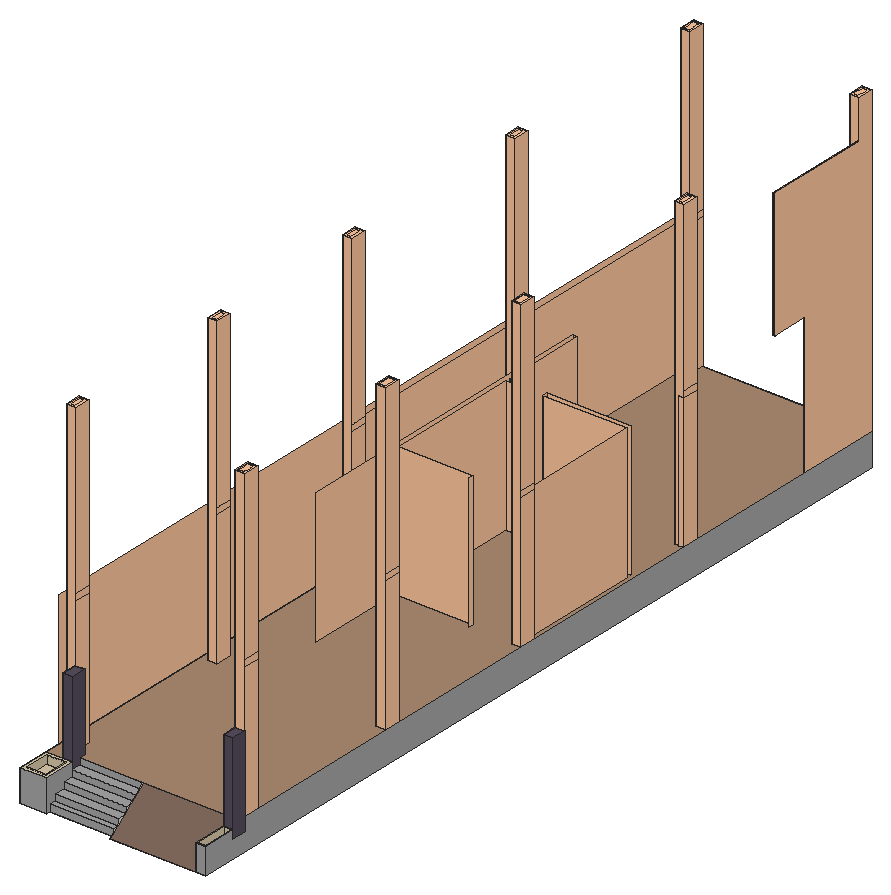
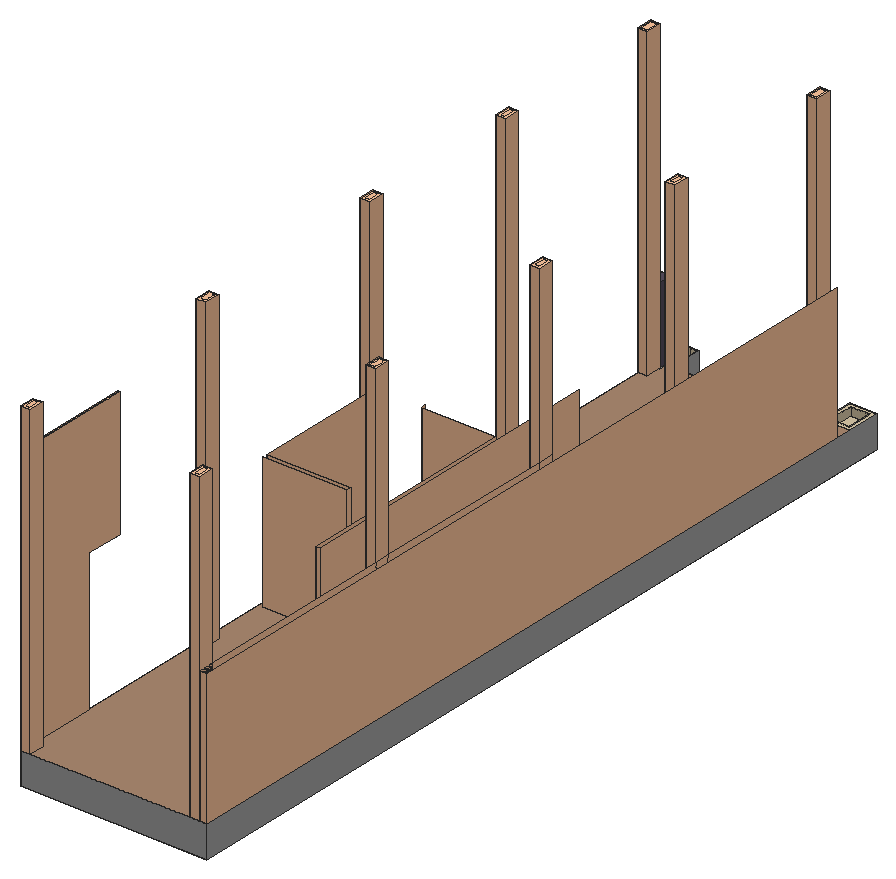
# SketchUp Ruby script. Lengths in inches.
U = 1.inch
M = Sketchup.active_model
def pt(a) = Geom::Point3d.new(a.map { |v| v * U })
def face(e, loops, mat)
  f = e.add_face(loops[0].map { |a| pt(a) })
  loops[1..].each { |l| e.add_face(l.map { |a| pt(a) }).erase! }
  f.material = f.back_material = mat if mat
  f
end
# faces: each face lists its corners as indices into pts; further lists are holes
def faces(e, pts, list, mat = nil) = list.each { |f| face(e, (f[0].is_a?(Array) ? f : [f]).map { |l| l.map { |i| pts[i] } }, mat) }
# xy, xz, yz: faces in a plane at the given z, y or x. An outline is a flat list of corners, or four numbers for a rectangle; further outlines are holes
def ring(l) = l.size == 4 ? [[l[0], l[1]], [l[2], l[1]], [l[2], l[3]], [l[0], l[3]]] : l.each_slice(2).to_a
def flat(e, list, mat, &to3) = list.each { |f| face(e, (f[0].is_a?(Array) ? f : [f]).map { |l| ring(l).map { |u, v| to3.(u, v) } }, mat) }
def xy(e, z, list, mat = nil) = flat(e, list, mat) { |x, y| [x, y, z] }
def xz(e, y, list, mat = nil) = flat(e, list, mat) { |x, z| [x, y, z] }
def yz(e, x, list, mat = nil) = flat(e, list, mat) { |y, z| [x, y, z] }
def lines(e, pts, list) = list.each { |a, b| e.add_line(pt(pts[a]), pt(pts[b])) }
# prism: a flat outline (further loops are holes) pulled along v
def prism(e, loops, v, mat = nil)
  f = face(e, loops, mat); d = Geom::Vector3d.new(v.map { |x| x * U })
  f.pushpull(f.normal.samedirection?(d) ? d.length : -d.length)
end
def box(e, o, s, mat = nil) = prism(e, [[o, [o[0] + s[0], o[1], o[2]], [o[0] + s[0], o[1] + s[1], o[2]], [o[0], o[1] + s[1], o[2]]]], [0, 0, s[2]], mat)
def at(x, y, z, deg = 0) = Geom::Transformation.translation(pt([x, y, z])) * Geom::Transformation.rotation(ORIGIN, Z_AXIS, deg.degrees)
def axes(o, x, y, z) = Geom::Transformation.new([*x, 0, *y, 0, *z, 0, *pt(o).to_a, 1])
def part(name) = M.definitions.add(name)
# library, detail: a bought-in or finely detailed component or shape, given as its bounding box
def library(name, o, s) = part(name).tap { |d| box(d.entities, o, s) }
def detail(e, o, s) = box(e.add_group.entities, o, s)
def put(e, d, t, mat = nil) = e.add_instance(d, t).tap { |i| i.material = mat if mat }
def group(e, t, mat = nil) = e.add_group.tap { |g| g.transformation = t; g.material = mat if mat }.entities
root = M.entities
M.materials.add("[0003_DeepPink]").color = [86, 78, 94]
M.materials.add("[Color A02]1").color = [252, 197, 157]
M.materials.add("[Field Square Tile]").color = [217, 201, 169]
M.materials.add("[Granite Brown]").color = [126, 104, 91]
M.materials.add("[Stone Vein Gray]").color = [166, 165, 165]
M.materials.add("[Tile Veriegated Stone]").color = [171, 137, 112]
c1 = part("Rectangular post")
box(c1.entities,[-0.01,0,-6],[8.99,13.95,85.25],"[0003_DeepPink]")
c2 = part("Rectangular post \#1")
box(c2.entities,[-0.01,0,-6],[8.99,13.95,78],"[0003_DeepPink]")
c3 = part("Structural column")
xy(c3.entities,0,[[[0,0.46,8.99,15.39],[2,2,7,13.17]]],"[Color A02]1")
xy(c3.entities,289.125,[[[0,0.46,8.99,15.39],[2,2,7,13.17]],[2,2,7,13.17]],"[Color A02]1")
xz(c3.entities,0.46,[[0,0,8.99,289.125]],"[Color A02]1")
xz(c3.entities,15.39,[[0,0,8.99,289.125]],"[Color A02]1")
yz(c3.entities,0,[[0.46,0,15.39,289.125]],"[Color A02]1")
yz(c3.entities,8.99,[[0.46,0,15.39,125.89],[0.46,125.89,15.39,131.89],[0.46,131.89,15.39,289.125]],"[Color A02]1")
p = [[7,2,0],[7,2,289.125],[2,2,0],[2,2,289.125],[7,13.17,0],[7,13.17,289.125],
  [2,13.17,0],[2,13.17,289.125]]
lines(c3.entities,p,[[0,1],[2,3],[4,5],[6,7]])
c4 = part("Wall section")
xy(c4.entities,0,[[[7.45,-62.8125,7.45,0.46,0,0.46,0,15.39,8.99,15.39,8.99,-62.8125],[2,2,7,13.17]]],"[Color A02]1")
xy(c4.entities,131.89,[[7.45,-98.7,8.98,-62.8125],[8.98,-98.7,8.99,-62.8125]],"[Color A02]1")
xy(c4.entities,251.89,[[7.45,-98.7,8.99,0.46]],"[Color A02]1")
xy(c4.entities,289.125,[[[0,0.46,8.99,15.39],[2,2,7,13.17]],[2,2,7,13.17]],"[Color A02]1")
xz(c4.entities,-98.7,[[7.45,131.89,8.99,251.89]],"[Color A02]1")
xz(c4.entities,-62.8125,[[7.45,0,8.99,131.89]],"[Color A02]1")
xz(c4.entities,0.46,[[0,0,7.45,0,7.45,251.89,8.99,251.89,8.99,289.125,0,289.125]],"[Color A02]1")
xz(c4.entities,15.39,[[0,0,8.99,289.125]],"[Color A02]1")
yz(c4.entities,0,[[0.46,0,15.39,289.125]],"[Color A02]1")
yz(c4.entities,7.45,[[-62.8125,0,-62.8125,131.89,-98.7,131.89,-98.7,251.89,0.46,251.89,0.46,0]],"[Color A02]1")
yz(c4.entities,8.99,[[-62.8125,0,15.39,0,15.39,289.125,0.46,289.125,0.46,251.89,-98.7,251.89,-98.7,131.89,-62.8125,131.89]],"[Color A02]1")
p = [[7,2,0],[7,2,289.125],[2,2,0],[2,2,289.125],[7,13.17,0],[7,13.17,289.125],
  [2,13.17,0],[2,13.17,289.125],[7.46,0.43,251.89],[8.99,0.43,251.89]]
lines(c4.entities,p,[[0,1],[2,3],[4,5],[6,7],[8,9]])
xy(root,-0.11,[[0.89,46.0625,7.86,784.43],[[7.86,371.24,16.85,386.1875],[8.87,372.26,8.87,378.59,9.5,377.95,10.39,377.07,11.28,376.18,12.13,377.04,13.01,376.14,13.89,377.02,13.01,377.92,13.89,378.8,14.77,379.67,15.65,380.55,15.83,380.36,15.83,378.97,15.65,378.78,13.89,377.02,14.77,376.13,15.65,375.23,14.77,374.36,15.65,373.46,15.83,373.27,15.83,372.26,15.2,372.26,14.82,372.64,13.93,373.52,13.05,372.64,12.16,373.52,13.05,374.41,12.16,375.3,11.28,374.41,12.16,373.52,11.28,372.64,10.39,373.52,9.5,372.64,9.12,372.26],[10.375,382.37,9.5,383.27,11.53,385.3,14.57,385.3,14.81,385.03,13.91,384.14,13.04,385.04,13.3,385.3,12.79,385.3,13.04,385.04,12.15,384.14,11.27,385.04,10.38,384.15,9.5,385.04,9.25,385.3,9.76,385.3,9.5,385.04,10.38,384.15,11.26,383.25],[12.13,382.36,11.26,383.25,12.15,384.14,13.02,383.25],[12.13,377.04,11.25,377.93,12.13,378.8125,13.01,377.92],[8.87,380.87,8.87,383.91,9.5,383.27,8.87,382.64,8.87,382.13,9.5,381.49],[15.65,384.11,14.81,385.03,15.07,385.3,15.83,385.3,15.83,384.29],[10.9,372.26,11.28,372.64,11.65,372.26,12.67,372.26,13.05,372.64,13.43,372.26],[15.83,375.04,15.65,375.23,15.83,375.42]],[8.87,372.26,9.12,372.26,9.5,372.64,8.87,373.27],[15.2,372.26,15.83,372.26,15.83,373.27,15.65,373.46,14.82,372.64],[9.5,372.64,10.39,373.52,9.5,374.41,8.87,373.78,8.87,373.27],
  [11.28,372.64,12.16,373.52,11.28,374.41,10.39,373.52],[13.05,372.64,13.93,373.52,13.05,374.41,12.16,373.52],[14.82,372.64,15.65,373.46,14.77,374.36,13.93,373.52],[15.83,373.27,15.83,373.65,15.65,373.46],[15.65,373.46,15.83,373.65,15.83,375.04,15.65,375.23,14.77,374.36],
  [10.39,373.52,11.28,374.41,12.16,375.3,10.39,377.07,9.5,377.95,10.375,378.83,9.5,379.72,8.87,379.09,8.87,380.36,9.5,379.72,10.375,378.83,11.25,379.71,12.13,380.58,11.25,381.48,10.375,380.6,11.25,379.71,10.375,378.83,11.25,377.93,8.87,375.55,8.87,375.04],[13.93,373.52,14.77,374.36,13.89,375.25,13.05,374.41],[8.87,373.78,9.5,374.41,8.87,375.04],[14.77,374.36,15.65,375.23,14.77,376.13,13.89,375.25],[13.05,374.41,13.89,375.25,13.01,376.14,12.16,375.3],
  [15.83,375.04,15.83,375.42,15.65,375.23],[171.33,375.17,171.33,375.42,171.21,375.3],[13.89,375.25,14.77,376.13,13.89,377.02,13.01,376.14],[12.16,375.3,13.01,376.14,12.13,377.04,11.28,376.18],[8.87,375.55,9.5,376.18,8.87,376.82],
  [9.5,376.18,10.39,377.07,9.5,377.95,8.87,377.32,8.87,376.82],[15.83,376.82,15.83,377.19,15.65,377.01],[171.33,376.88,171.33,377.19,171.18,377.04],[15.65,377.01,15.83,377.19,15.83,378.59,15.65,378.78,14.77,377.9],[13.89,377.02,14.77,377.9,13.89,378.8,13.01,377.92],
  [12.13,377.04,13.01,377.92,12.13,378.8125,11.25,377.93],[171.18,377.04,171.33,377.19,171.33,378.65,171.18,378.8125,170.3,377.93],[10.39,377.07,11.25,377.93,10.375,378.83,9.5,377.95],[8.87,377.32,9.5,377.95,8.87,378.59],[14.77,377.9,15.65,378.78,14.77,379.67,13.89,378.8],
  [171.33,378.65,171.33,378.97,171.18,378.8125],[15.65,378.78,15.83,378.97,15.83,380.36,15.65,380.55,14.77,379.67],[12.13,378.8125,13.01,379.69,12.13,380.58,11.25,381.48,10.375,382.37,9.5,381.49,11.25,379.71],[12.13,378.8125,13.01,379.69,12.13,380.58,11.25,379.71],[171.18,378.8125,171.33,378.97,171.33,380.43,171.18,380.58,170.3,379.71],
  [8.87,379.09,9.5,379.72,8.87,380.36],[13.01,379.69,13.89,380.57,13.01,381.46,12.13,380.58],[13.01,379.69,15.65,382.33,14.78,383.23,13.91,384.14,13.02,383.25,13.9,382.35,14.78,383.23,15.65,384.11,15.83,384.29,15.83,385.3,15.07,385.3,14.81,385.03,15.65,384.11,14.78,383.23,13.9,382.35,14.77,381.45,13.9,382.35,12.13,380.58],[171.33,380.43,171.33,380.74,171.18,380.58],[15.65,380.55,15.83,380.74,15.83,382.13,15.65,382.33,15.83,382.51,15.83,382.13,15.65,382.33,14.78,383.23,13.9,382.35,14.77,381.45],
  [15.65,380.55,15.83,380.74,15.83,382.13,15.65,382.33,14.77,381.45],[13.89,380.57,14.77,381.45,13.9,382.35,13.01,381.46],[12.13,380.58,13.01,381.46,12.13,382.36,11.25,381.48],[10.375,380.6,11.25,381.48,10.375,382.37,9.5,381.49],[8.87,380.87,9.5,381.49,8.87,382.13],
  [15.83,382.13,15.83,382.51,15.65,382.33],[13.9,382.35,14.78,383.23,13.91,384.14,13.02,383.25],[12.13,382.36,13.02,383.25,12.15,384.14,11.26,383.25],[10.375,382.37,11.26,383.25,10.38,384.15,9.5,383.27],[8.87,382.64,9.5,383.27,8.87,383.91],
  [15.65,384.11,15.83,384.29,15.83,385.3,15.07,385.3,14.81,385.03],[12.15,384.14,13.04,385.04,12.79,385.3,11.53,385.3,11.27,385.04],[13.91,384.14,14.81,385.03,14.57,385.3,13.3,385.3,13.04,385.04],[9.5,385.04,9.76,385.3,9.25,385.3],[[7.86,563.34,16.85,578.28],[8.87,564.35,8.87,565.36,9.5,564.73,9.12,564.35,9.88,564.35,9.5,564.73,10.39,565.62,9.5,566.5,8.87,567.14,8.87,567.64,9.5,568.28,10.39,567.39,9.5,566.5,10.39,565.62,11.28,566.5,10.39,567.39,11.28,568.28,10.39,569.16,9.5,570.05,10.375,570.92,9.5,571.81,8.87,571.1875,8.87,570.68,9.5,570.05,8.87,569.42,8.87,577.27,14.57,577.27,14.82,577.02,13.92,576.14,14.76,575.3,13.87,574.42,13.03,575.26,13.92,576.14,13.04,577.02,13.3,577.27,12.79,577.27,13.04,577.02,12.14,576.14,11.27,577.02,11.53,577.27,11.02,577.27,11.27,577.02,10.36,576.16,9.45,575.29,10.35,574.4,11.24,573.51,10.34,572.63,9.45,573.52,10.35,574.4,9.45,575.29,8.87,574.73,8.87,574.1,9.45,573.52,8.87,572.96,8.87,572.46,9.5,571.81,11.25,570.03,10.39,569.16,11.28,568.28,12.13,569.13,11.25,570.03,12.1,570.87,12.98,569.99,13.87,570.87,12.98,571.76,13.87,572.65,14.76,571.76,13.87,570.87,12.98,569.99,14.76,568.21,15.64,569.1,15.83,569.29,15.83,567.14,15.64,567.33,14.77,566.45,13.93,565.62,13.05,566.5,12.16,565.62,13.05,564.73,12.67,564.35,13.43,564.35,13.05,564.73,13.93,565.62,14.82,564.73,14.44,564.35],[12.1,570.87,11.21,571.76,12.1,572.65,12.98,571.76]],
  [8.87,564.35,9.12,564.35,9.5,564.73,8.87,565.36],[9.88,564.35,10.9,564.35,11.28,564.73,10.39,565.62,9.5,564.73],[10.9,564.35,11.65,564.35,11.28,564.73,12.16,565.62,11.28,566.5,10.39,565.62,11.28,564.73],[11.65,564.35,12.67,564.35,13.05,564.73,12.16,565.62,11.28,564.73],[13.43,564.35,14.44,564.35,14.82,564.73,13.93,565.62,13.05,564.73],
  [15.2,564.35,15.83,564.35,15.83,565.36,15.65,565.56,14.82,564.73],[15.2,564.35,15.83,564.35,15.83,565.74,14.82,564.73],[9.5,564.73,10.39,565.62,9.5,566.5,8.87,565.87,8.87,565.36],[15.83,565.36,15.83,565.74,15.65,565.56,14.77,566.45,15.64,567.33,14.76,568.21,13.89,567.34,13.01,568.24,12.16,567.39,13.05,566.5,13.89,567.34,15.65,565.56],[12.16,565.62,13.05,566.5,12.16,567.39,11.28,566.5],
  [13.93,565.62,14.77,566.45,13.89,567.34,13.05,566.5],[8.87,565.87,9.5,566.5,8.87,567.14],[173.8125,566.45,174.6875,567.33,173.8,568.21,172.93,567.34],[9.5,566.5,10.39,567.39,9.5,568.28,8.87,567.64,8.87,567.14],[11.28,566.5,12.16,567.39,11.28,568.28,10.39,567.39],
  [15.83,567.14,15.83,567.52,15.64,567.33],[15.64,567.33,15.83,567.52,15.83,568.91,15.64,569.1,14.76,568.21],[13.89,567.34,14.76,568.21,13.87,569.1,13.01,568.24],[172.93,567.34,173.8,568.21,172.92,569.1,172.06,568.24],[12.16,567.39,13.01,568.24,12.13,569.13,11.28,568.28],
  [171.21,567.39,172.06,568.24,171.33,568.97,171.18,569.13,170.32,568.28],[173.8,568.21,174.6875,569.1,173.8,569.99,172.92,569.1],[13.01,568.24,13.87,569.1,12.98,569.99,12.13,569.13],[172.06,568.24,172.92,569.1,172.03,569.99,171.33,569.29,171.33,568.97],[15.83,568.91,15.83,569.29,15.64,569.1],
  [172.92,569.1,173.8,569.99,172.92,570.87,172.03,569.99],[12.13,569.13,12.98,569.99,12.1,570.87,11.25,570.03],[10.39,569.16,11.25,570.03,10.375,570.92,9.5,570.05],[8.87,569.42,9.5,570.05,8.87,570.68],[173.8,569.99,174.6875,570.87,173.8,571.76,172.92,570.87],
  [12.1,570.87,12.98,571.76,12.1,572.65,11.21,571.76],[13.87,570.87,14.76,571.76,13.87,572.65,12.98,571.76],[15.64,570.87,15.83,571.0625,15.83,577.27,15.07,577.27,14.82,577.02,15.64,576.19,15.83,576.38,15.83,576,15.64,576.19,14.76,575.3,13.87,574.42,13.03,575.26,13.92,576.14,15.64,574.42,15.83,574.61,15.83,574.23,15.64,574.42,14.76,573.53,15.64,572.65,15.83,572.84,15.83,572.46,15.64,572.65,14.76,571.76],[15.64,570.87,15.83,571.0625,15.83,572.46,15.64,572.65,14.76,571.76],[172.92,570.87,173.8,571.76,172.92,572.65,172.03,571.76],
  [10.375,570.92,11.21,571.76,10.34,572.63,11.21,571.76,12.1,572.65,11.24,573.51,10.34,572.63,9.5,571.81,8.87,572.46,8.87,571.1875,9.5,571.81],[10.375,570.92,11.21,571.76,10.34,572.63,9.5,571.81],[8.87,571.1875,9.5,571.81,8.87,572.46],[11.21,571.76,12.1,572.65,11.24,573.51,10.34,572.63],[10.34,572.63,11.24,573.51,10.35,574.4,9.45,573.52],
  [12.1,572.65,12.98,573.53,12.13,574.38,11.24,573.51],[12.1,572.65,13.87,574.42,13.03,575.26,12.13,574.38,11.24,573.51],[13.87,572.65,14.76,573.53,13.03,575.26,12.14,576.14,11.25,575.27,12.13,574.38,12.98,573.53],[13.87,572.65,14.76,573.53,13.87,574.42,12.98,573.53],[15.64,572.65,15.83,572.84,15.83,574.23,15.64,574.42,14.76,573.53],
  [8.87,572.96,9.45,573.52,8.87,574.1],[12.13,574.38,13.03,575.26,12.14,576.14,11.25,575.27],[15.64,574.42,15.83,574.61,15.83,576,15.64,576.19,14.76,575.3],[8.87,574.73,9.45,575.29,8.87,575.875],[9.45,575.29,10.36,576.16,9.48,577.03,9.76,577.27,9.25,577.27,9.48,577.03,8.87,576.51,8.87,575.875],
  [12.14,576.14,13.04,577.02,12.79,577.27,11.53,577.27,11.27,577.02],[13.92,576.14,14.82,577.02,14.57,577.27,13.3,577.27,13.04,577.02],[10.36,576.16,11.27,577.02,11.02,577.27,9.76,577.27,9.48,577.03],[15.64,576.19,15.83,576.38,15.83,577.27,15.07,577.27,14.82,577.02],[8.87,576.51,9.48,577.03,9.25,577.27,8.87,577.27],
  [[7.86,769.36,16.85,784.43],[8.87,771.89,8.87,778.48,11.28,776.07,12.16,775.1875,13.05,776.07,13.93,775.1875,13.05,774.3,11.28,772.53,10.39,773.41,9.5,772.53],[15.71,776.96,14.82,777.85,15.71,778.73,15.83,778.61,15.83,778.86,15.71,778.73,13.93,780.51,14.78,781.35,15.65,782.22,14.81,783.15,14.57,783.42,15.07,783.42,14.81,783.15,15.65,782.22,15.83,782.02,15.83,777.09],[11.27,770.76,10.39,771.64,11.28,772.53,12.15,771.66],[15.65,775.25,14.82,776.07,15.71,776.96,15.83,776.83,15.83,775.44],[8.87,780.76,8.87,782.02,9.5,781.39],[14.44,770.375,14.8,770.77,15.2,770.375],[12.67,770.375,13.04,770.76,13.43,770.375],[10.9,770.375,11.27,770.76,11.65,770.375],[9.12,770.375,9.5,770.75,9.88,770.375],[15.83,771.51,15.65,771.7,15.83,771.89]],[8.87,770.375,9.12,770.375,9.5,770.75,10.39,771.64,11.27,770.76,12.15,771.66,13.04,770.76,12.67,770.375,11.65,770.375,11.27,770.76,10.9,770.375,15.2,770.375,14.8,770.77,14.44,770.375,13.43,770.375,13.04,770.76,13.91,771.67,14.8,770.77,15.65,771.7,14.78,772.57,15.65,773.47,15.83,773.29,15.83,775.44,15.65,775.25,15.83,775.06,15.83,773.67,15.65,773.47,14.77,774.35,15.65,775.25,14.82,776.07,15.71,776.96,14.82,777.85,13.93,776.96,13.05,777.85,12.16,778.73,13.05,779.62,12.16,780.51,11.28,779.62,10.39,780.51,9.5,779.62,8.87,780.25,8.87,778.99,10.39,780.51,11.28,781.39,12.16,782.28,13.04,783.16,12.79,783.42,11.53,783.42,11.28,783.16,10.39,782.28,9.5,783.16,9.76,783.42,9.25,783.42,9.5,783.16,10.39,782.28,9.5,781.39,10.39,780.51,11.28,779.62,12.16,778.73,13.05,777.85,12.16,776.96,11.28,776.07,12.16,775.1875,11.28,774.3,10.39,775.1875,11.28,776.07,12.16,776.96,13.05,776.07,13.93,776.96,14.82,776.07,13.93,775.1875,14.77,774.35,15.65,773.47,13.91,771.67,13.04,770.76,12.15,771.66,11.28,772.53,9.5,770.75,8.87,771.39],[8.87,770.375,9.12,770.375,9.5,770.75,8.87,771.39],[9.12,770.375,9.88,770.375,9.5,770.75],[10.9,770.375,11.65,770.375,11.27,770.76],
  [12.67,770.375,13.43,770.375,13.04,770.76],[14.44,770.375,15.2,770.375,14.8,770.77],[11.27,770.76,12.15,771.66,11.28,772.53,10.39,771.64],[14.8,770.77,15.65,771.7,14.78,772.57,13.91,771.67],[15.83,771.51,15.83,771.89,15.65,771.7],
  [8.87,771.89,9.5,772.53,8.87,773.16],[9.5,772.53,10.39,773.41,9.5,774.3,8.87,773.67,8.87,773.16],[11.28,772.53,12.16,773.41,11.28,774.3,10.39,773.41],[15.83,773.29,15.83,773.67,15.65,773.47],[10.39,773.41,11.28,774.3,10.39,775.1875,9.5,776.07,10.39,776.96,9.5,777.85,8.87,777.21,8.87,776.71,9.5,776.07,8.87,775.44,8.87,774.93],
  [12.16,773.41,13.05,774.3,12.16,775.1875,11.28,774.3],[8.87,773.67,9.5,774.3,8.87,774.93],[11.28,774.3,12.16,775.1875,11.28,776.07,10.39,775.1875],[13.05,774.3,13.93,775.1875,13.05,776.07,12.16,775.1875],[14.77,774.35,15.65,775.25,14.82,776.07,13.93,775.1875],
  [15.83,775.06,15.83,775.44,15.65,775.25],[10.39,775.1875,11.28,776.07,10.39,776.96,9.5,776.07],[15.65,775.25,15.83,775.44,15.83,776.83,15.71,776.96,14.82,776.07],[8.87,775.44,9.5,776.07,8.87,776.71],[13.05,776.07,13.93,776.96,13.05,777.85,12.16,776.96],
  [14.82,776.07,15.71,776.96,14.82,777.85,13.93,776.96],[10.39,776.96,11.28,777.85,10.39,778.73,9.5,777.85],[10.39,776.96,11.28,777.85,10.39,778.73,9.5,777.85],[15.71,776.96,15.83,777.09,15.83,782.02,15.65,782.22,14.81,783.15,15.07,783.42,14.57,783.42,14.81,783.15,15.65,782.22,14.78,781.35,13.93,780.51,15.71,778.73,15.83,778.86,15.83,778.61,15.71,778.73,14.82,777.85],[15.71,776.96,15.83,777.09,15.83,778.61,15.71,778.73,14.82,777.85],
  [8.87,777.21,9.5,777.85,8.87,778.48],[11.28,777.85,12.16,778.73,13.05,777.85,14.82,779.62,13.05,781.39,12.16,780.51,13.05,779.62,13.93,780.51,14.78,781.35,15.65,780.45,15.83,780.63,15.83,780.25,15.65,780.45,13.93,778.73,13.05,779.62,11.28,777.85,10.39,778.73,11.28,779.62,12.16,780.51,11.28,781.39,10.39,780.51,11.28,779.62,10.39,778.73],[13.05,777.85,13.93,778.73,13.05,779.62,12.16,778.73],[12.16,778.73,13.05,779.62,12.16,780.51,11.28,779.62],[15.71,778.73,15.83,778.86,15.83,780.25,15.65,780.45,14.82,779.62],
  [8.87,778.99,9.5,779.62,8.87,780.25],[11.28,779.62,12.16,780.51,11.28,781.39,10.39,780.51],[13.05,779.62,13.93,780.51,13.05,781.39,12.16,780.51],[14.82,779.62,15.65,780.45,14.78,781.35,13.93,780.51],[15.65,780.45,15.83,780.63,15.83,782.02,15.65,782.22,14.78,781.35],
  [10.39,780.51,11.28,781.39,10.39,782.28,9.5,781.39],[8.87,780.76,9.5,781.39,8.87,782.02],[11.28,781.39,12.16,782.28,11.28,783.16,10.39,782.28],[12.16,782.28,13.04,783.16,12.79,783.42,11.53,783.42,11.28,783.16],[14.81,783.15,15.07,783.42,14.57,783.42],
  [9.5,783.16,9.76,783.42,9.25,783.42]],"[Color A02]1")
xz(root,375.68,[[57.37,-0.11,126.89,125.89]],"[Color A02]1")
xz(root,501.8,[[57.37,-0.11,63.32,125.89],[92.32,-0.11,171.33,125.89]],"[Color A02]1")
xz(root,506.23,[[57.37,-0.11,63.32,125.89],[92.32,-0.11,171.33,125.89]],"[Color A02]1")
xz(root,563.34,[[171.33,-0.11,175.89,125.89]],"[Color A02]1")
xz(root,585.88,[[52.81,-0.11,57.37,125.89]],"[Color A02]1")
xz(root,784.43,[[0.89,-0.11,7.86,125.89]],"[Color A02]1")
yz(root,0.89,[[46.0625,-0.11,784.43,125.89]],"[Color A02]1")
yz(root,7.86,[[371.24,-0.11,386.1875,125.89],[386.1875,-0.11,563.34,125.89],[563.34,-0.11,578.28,125.89],[578.28,-0.11,769.36,125.89],[769.36,-0.11,784.43,125.89]],"[Color A02]1")
yz(root,52.81,[[283.24,-0.11,585.88,125.89]],"[Color A02]1")
yz(root,57.37,[[375.68,-0.11,501.8,125.89],[506.23,-0.11,585.88,125.89]],"[Color A02]1")
yz(root,63.32,[[501.8,-0.11,506.23,125.89]],"[Color A02]1")
yz(root,92.32,[[501.8,-0.11,506.23,125.89]],"[Color A02]1")
yz(root,126.89,[[371.24,-0.11,375.68,125.89]],"[Color A02]1")
yz(root,171.33,[[386.1875,-0.11,501.8,125.89]],"[Color A02]1")
g1 = group(root,at(0.91,46.0625,-6))
xy(g1,-24,[[0,-46.0625,0,738.37,175,738.37,175,-46.0625,84.9375,-46.0625,84.9375,-42.1875,24.9375,-42.1875,24.9375,-46.0625]])
xy(g1,-18,[[24.9375,-42.1875,84.9375,-36.0625]],"[Stone Vein Gray]")
xy(g1,-17.375,[[166.8,-45.26,174.2,-14.76]],"[Field Square Tile]")
xy(g1,-12,[[24.9375,-36.0625,84.9375,-26.0625]],"[Stone Vein Gray]")
xy(g1,-7.25,[[165.99,-13.95,175,0.05]])
xy(g1,-6,[[24.9375,-26.0625,84.9375,-16.33]],"[Stone Vein Gray]")
xy(g1,-1.875,[[3.35,-42.71,21.58,-18.47]],"[Field Square Tile]")
xy(g1,0,[[15.95,-15.11,24.9375,-0.84]],"[Field Square Tile]")
xy(g1,0,[[24.9375,-16.33,84.9375,-7.14]],"[Stone Vein Gray]")
xy(g1,0.75,[[[165.99,-46.0625,175,-13.95],[166.8,-45.26,174.2,-14.76]]],"[Field Square Tile]")
xy(g1,6,[[[0,-46.0625,24.9375,-15.11],[3.35,-42.71,21.58,-18.47]]],"[Field Square Tile]")
xy(g1,6,[[0,-15.11,15.95,-15.11,15.95,-0.84,24.9375,-0.84,24.9375,-7.14,165.99,-7.14,165.99,0,175,0,175,738.37,0,738.37]],"[Tile Veriegated Stone]")
xz(g1,-46.0625,[[0,-24,24.9375,6],[165.99,-24,175,0.75]],"[Stone Vein Gray]")
xz(g1,-45.26,[[166.8,-17.375,174.2,0.75]],"[Field Square Tile]")
xz(g1,-42.71,[[3.35,-1.875,21.58,6]],"[Field Square Tile]")
xz(g1,-42.1875,[[24.9375,-24,84.9375,-18]],"[Stone Vein Gray]")
xz(g1,-36.0625,[[24.9375,-18,84.9375,-12]],"[Stone Vein Gray]")
xz(g1,-26.0625,[[24.9375,-12,84.9375,-6]],"[Stone Vein Gray]")
xz(g1,-18.47,[[3.35,-1.875,21.58,6]],"[Field Square Tile]")
xz(g1,-16.33,[[24.9375,-6,84.9375,0]],"[Stone Vein Gray]")
xz(g1,-15.11,[[15.95,0,24.9375,6]],"[Field Square Tile]")
xz(g1,-14.76,[[166.8,-17.375,174.2,0.75]],"[Field Square Tile]")
xz(g1,-13.95,[[165.99,-7.25,175,0.75]])
xz(g1,-7.14,[[24.9375,0,84.9375,6]],"[Stone Vein Gray]")
xz(g1,-0.84,[[15.95,0,24.9375,6]],"[Field Square Tile]")
xz(g1,0,[[165.99,5.89,175,6]])
xz(g1,0.05,[[165.99,-7.25,175,0.75]])
xz(g1,738.37,[[0,-24,175,6]],"[Stone Vein Gray]")
yz(g1,0,[[-46.0625,-24,738.37,6]],"[Stone Vein Gray]")
yz(g1,3.35,[[-42.71,-1.875,-18.47,6]],"[Field Square Tile]")
yz(g1,15.95,[[-15.11,0,-14.28,6],[-14.28,0,-0.84,6],[-0.84,0,-0.56,6]],"[Field Square Tile]")
yz(g1,21.58,[[-42.71,-1.875,-18.47,6]],"[Field Square Tile]")
yz(g1,24.9375,[[-7.14,0,-0.84,6]],"[Field Square Tile]")
yz(g1,24.9375,[[-46.0625,-24,-42.1875,-24,-42.1875,-18,-36.0625,-18,-36.0625,-12,-26.0625,-12,-26.0625,-6,-16.33,-6,-16.33,0,-15.11,0,-15.11,6,-46.0625,6]],"[Stone Vein Gray]")
yz(g1,84.9375,[[-46.0625,-24,-42.1875,-21.01,-38.28,-18,-36.0625,-16.29,-30.49,-12,-26.0625,-8.59,-22.71,-6,-16.33,-1.08,-14.92,0,-7.14,6,-7.14,0,-16.33,0,-16.33,-6,-26.0625,-6,-26.0625,-12,-36.0625,-12,-36.0625,-18,-42.1875,-18,-42.1875,-24]])
yz(g1,165.99,[[-13.95,-7.25,0.05,-7.25,0.05,0.75,0,5.89,0,6,-7.14,6,-13.95,0.75]])
yz(g1,165.99,[[-46.0625,-24,-46.0625,0.75,-13.95,0.75]],"[Stone Vein Gray]")
yz(g1,166.8,[[-45.26,-17.375,-14.76,0.75]],"[Field Square Tile]")
yz(g1,174.2,[[-45.26,-17.375,-14.76,0.75]],"[Field Square Tile]")
yz(g1,175,[[-46.0625,-24,738.37,-24,738.37,6,0,6,0,5.89,0.05,0.75,0.05,-7.25,-13.95,-7.25,-13.95,0.75,-46.0625,0.75]],"[Stone Vein Gray]")
p = [[84.9375,-46.0625,-24],[165.99,-46.0625,-24],[165.99,-13.95,0.75],[165.99,-7.14,6],[164.99,-7.14,6],[84.9375,-7.14,6],
  [84.9375,-14.92,0],[84.9375,-16.33,-1.08],[84.9375,-22.71,-6],[84.9375,-26.0625,-8.59],[84.9375,-30.49,-12],[84.9375,-36.0625,-16.29],
  [84.9375,-38.28,-18],[84.9375,-42.1875,-21.01],[175,0.05,0.75],[175,0,5.89],[165.99,0,5.89],[165.99,0.05,0.75],
  [15.95,14.93,5.89],[165.99,15.07,5.89],[166.01,-14.23,0.75],[-0.02,-15.11,6],[0,-15.11,6]]
faces(g1,p,[[0,1,2,3,4,5,6,7,8,9,10,11,12,13]],"[Granite Brown]")
faces(g1,p,[[14,15,16,17]])
lines(g1,p,[[18,19],[20,1],[21,22]])
put(g1,c1,at(166.02,-13.95,-1.25))
put(g1,c2,at(15.96,-15.11,6))
g2 = group(root,at(7.86,46.0625,-0.11))
p = [[168.04,0,126],[168.04,0,132]]
lines(g2,p,[[0,1]])
put(g2,c3,at(0.01,165.91,0.11))
put(g2,c3,at(159.04,-0.46,0.11),"[Color A02]1")
put(g2,c3,at(0,-0.46,0))
put(g2,c3,at(0.01,324.73,0.11))
put(g2,c3,at(0.01,516.83,0.11))
put(g2,c3,at(0,722.98,0.13))
put(g2,c4,at(159.05,722.98,0.11))
put(g2,c3,at(159.04,324.73,0.11))
put(g2,c3,at(159.04,516.83,0.11))
put(g2,c3,at(159.04,165.6875,0.11))
